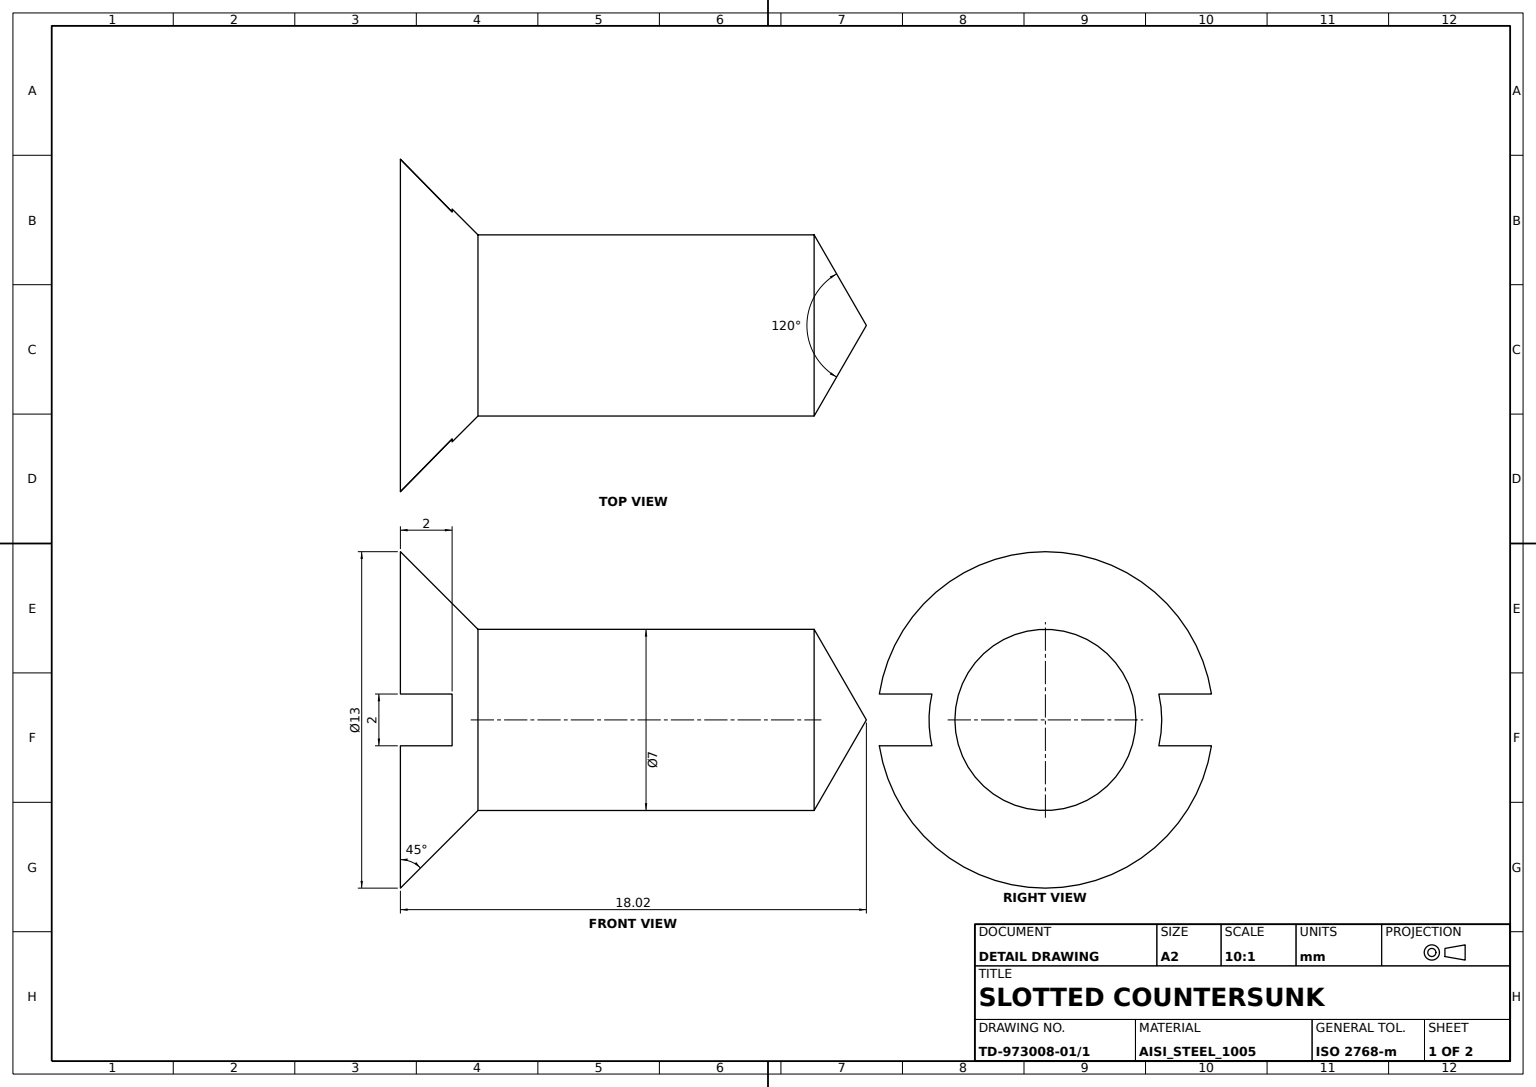
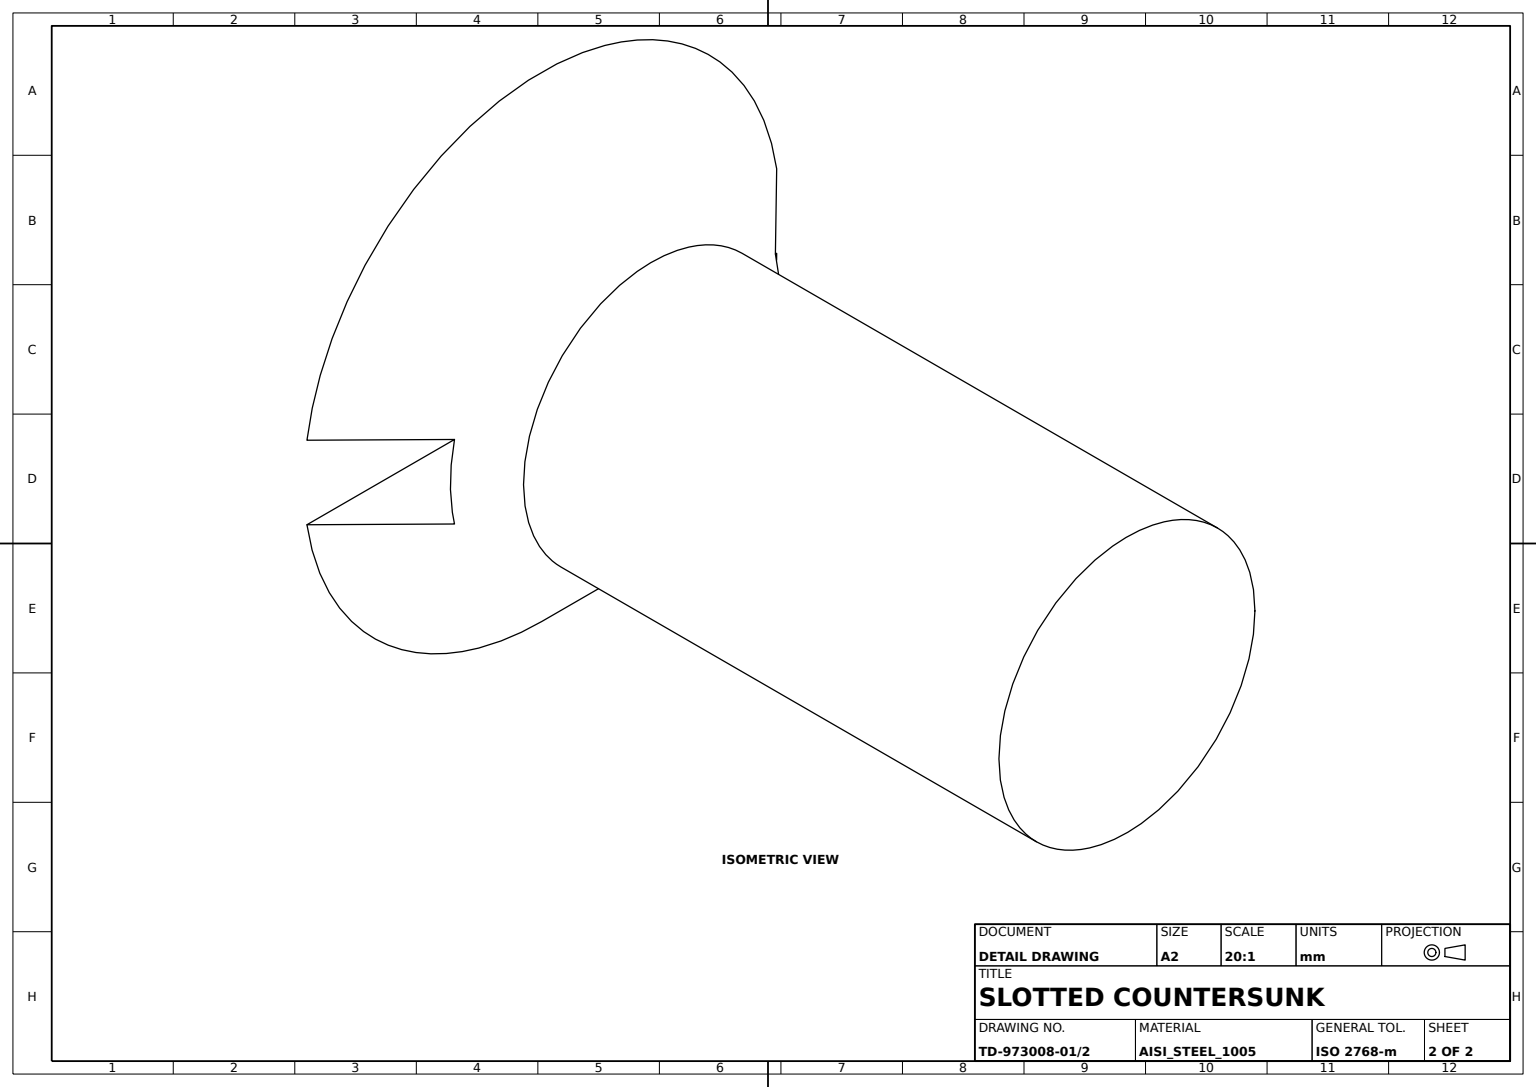
ISO-10303-21;
HEADER;
FILE_DESCRIPTION((''),'2;1');
FILE_NAME('','',(''),(''),'','','');
FILE_SCHEMA(('AUTOMOTIVE_DESIGN'));
ENDSEC;
DATA;
#1=APPLICATION_CONTEXT('');
#2=PRODUCT_CONTEXT('',#1,'mechanical');
#3=PRODUCT('','','',(#2));
#4=PRODUCT_DEFINITION_FORMATION('','',#3);
#5=PRODUCT_DEFINITION_CONTEXT('',#1,'design');
#6=PRODUCT_DEFINITION('','',#4,#5);
#7=PRODUCT_DEFINITION_SHAPE('','',#6);
#8=(LENGTH_UNIT()NAMED_UNIT(*)SI_UNIT(.MILLI.,.METRE.));
#9=(NAMED_UNIT(*)PLANE_ANGLE_UNIT()SI_UNIT($,.RADIAN.));
#10=(NAMED_UNIT(*)SI_UNIT($,.STERADIAN.)SOLID_ANGLE_UNIT());
#11=UNCERTAINTY_MEASURE_WITH_UNIT(LENGTH_MEASURE(0.005),#8,'distance_accuracy_value','');
#12=(GEOMETRIC_REPRESENTATION_CONTEXT(3)GLOBAL_UNCERTAINTY_ASSIGNED_CONTEXT((#11))GLOBAL_UNIT_ASSIGNED_CONTEXT((#8,#9,#10))REPRESENTATION_CONTEXT('',''));
#13=CARTESIAN_POINT('',(-17.425463,-1.,6.422616));
#14=VERTEX_POINT('',#13);
#15=CARTESIAN_POINT('',(-17.425463,-1.,-6.422616));
#16=VERTEX_POINT('',#15);
#17=CARTESIAN_POINT('',(-17.425463,-1.,7.));
#18=DIRECTION('',(0.,0.,-1.));
#19=VECTOR('',#18,1000.);
#20=LINE('',#17,#19);
#21=EDGE_CURVE('',#14,#16,#20,.T.);
#22=ORIENTED_EDGE('',*,*,#21,.T.);
#23=CARTESIAN_POINT('',(-17.425463,0.,0.));
#24=DIRECTION('',(1.,0.,0.));
#25=AXIS2_PLACEMENT_3D('',#23,#24,#18);
#26=CIRCLE('',#25,6.5);
#27=EDGE_CURVE('',#14,#16,#26,.T.);
#28=ORIENTED_EDGE('',*,*,#27,.F.);
#29=EDGE_LOOP('',(#22,#28));
#30=FACE_BOUND('',#29,.T.);
#31=CARTESIAN_POINT('',(-17.425463,6.5,0.));
#32=DIRECTION('',(-1.,0.,0.));
#33=DIRECTION('',(0.,0.,1.));
#34=AXIS2_PLACEMENT_3D('',#31,#32,#33);
#35=PLANE('',#34);
#36=ADVANCED_FACE('',(#30),#35,.T.);
#37=ORIENTED_EDGE('',*,*,#27,.T.);
#38=CARTESIAN_POINT('',(-15.425463,-1.,-4.387482));
#39=VERTEX_POINT('',#38);
#40=CARTESIAN_POINT('',(-16.089461,-1.,-5.068508));
#41=CARTESIAN_POINT('',(-16.756961,-1.,-5.746059));
#42=B_SPLINE_CURVE_WITH_KNOTS('',3,(#38,#40,#41,#15),.UNSPECIFIED.,.F.,.F.,(4,4),(0.025452548,0.028328148),.UNSPECIFIED.);
#43=EDGE_CURVE('',#39,#16,#42,.T.);
#44=ORIENTED_EDGE('',*,*,#43,.F.);
#45=CARTESIAN_POINT('',(-15.425463,1.,-4.387482));
#46=VERTEX_POINT('',#45);
#47=CARTESIAN_POINT('',(-15.425463,0.,0.));
#48=AXIS2_PLACEMENT_3D('',#47,#24,#18);
#49=CIRCLE('',#48,4.5);
#50=EDGE_CURVE('',#46,#39,#49,.F.);
#51=ORIENTED_EDGE('',*,*,#50,.F.);
#52=CARTESIAN_POINT('',(-17.425463,1.,-6.422616));
#53=VERTEX_POINT('',#52);
#54=CARTESIAN_POINT('',(-16.756955,1.,-5.746054));
#55=CARTESIAN_POINT('',(-16.089453,1.,-5.0685));
#56=B_SPLINE_CURVE_WITH_KNOTS('',3,(#52,#54,#55,#45),.UNSPECIFIED.,.F.,.F.,(4,4),(0.011190983,0.014044358),.UNSPECIFIED.);
#57=EDGE_CURVE('',#53,#46,#56,.T.);
#58=ORIENTED_EDGE('',*,*,#57,.F.);
#59=CARTESIAN_POINT('',(-17.425463,1.,6.422616));
#60=VERTEX_POINT('',#59);
#61=EDGE_CURVE('',#53,#60,#26,.T.);
#62=ORIENTED_EDGE('',*,*,#61,.T.);
#63=CARTESIAN_POINT('',(-15.425463,1.,4.387482));
#64=VERTEX_POINT('',#63);
#65=CARTESIAN_POINT('',(-16.089461,1.,5.068508));
#66=CARTESIAN_POINT('',(-16.756961,1.,5.746059));
#67=B_SPLINE_CURVE_WITH_KNOTS('',3,(#63,#65,#66,#59),.UNSPECIFIED.,.F.,.F.,(4,4),(0.025452548,0.028328148),.UNSPECIFIED.);
#68=EDGE_CURVE('',#64,#60,#67,.T.);
#69=ORIENTED_EDGE('',*,*,#68,.F.);
#70=CARTESIAN_POINT('',(-15.425463,-1.,4.387482));
#71=VERTEX_POINT('',#70);
#72=EDGE_CURVE('',#71,#64,#49,.F.);
#73=ORIENTED_EDGE('',*,*,#72,.F.);
#74=CARTESIAN_POINT('',(-16.756955,-1.,5.746054));
#75=CARTESIAN_POINT('',(-16.089453,-1.,5.0685));
#76=B_SPLINE_CURVE_WITH_KNOTS('',3,(#13,#74,#75,#70),.UNSPECIFIED.,.F.,.F.,(4,4),(0.011190983,0.014044358),.UNSPECIFIED.);
#77=EDGE_CURVE('',#14,#71,#76,.T.);
#78=ORIENTED_EDGE('',*,*,#77,.F.);
#79=EDGE_LOOP('',(#37,#44,#51,#58,#62,#69,#73,#78));
#80=FACE_BOUND('',#79,.T.);
#81=CARTESIAN_POINT('',(-14.425463,0.,-3.5));
#82=VERTEX_POINT('',#81);
#83=CARTESIAN_POINT('',(-14.425463,0.,0.));
#84=AXIS2_PLACEMENT_3D('',#83,#24,#18);
#85=CIRCLE('',#84,3.5);
#86=EDGE_CURVE('',#82,#82,#85,.T.);
#87=ORIENTED_EDGE('',*,*,#86,.F.);
#88=EDGE_LOOP('',(#87));
#89=FACE_BOUND('',#88,.T.);
#90=AXIS2_PLACEMENT_3D('',#83,#32,#33);
#91=CONICAL_SURFACE('',#90,3.5,0.785398163);
#92=ADVANCED_FACE('',(#80,#89),#91,.T.);
#93=ORIENTED_EDGE('',*,*,#21,.F.);
#94=ORIENTED_EDGE('',*,*,#77,.T.);
#95=CARTESIAN_POINT('',(-15.425463,-1.,7.));
#96=LINE('',#95,#19);
#97=EDGE_CURVE('',#39,#71,#96,.F.);
#98=ORIENTED_EDGE('',*,*,#97,.F.);
#99=ORIENTED_EDGE('',*,*,#43,.T.);
#100=EDGE_LOOP('',(#93,#94,#98,#99));
#101=FACE_BOUND('',#100,.T.);
#102=DIRECTION('',(0.,-1.,0.));
#103=AXIS2_PLACEMENT_3D('',#95,#102,#24);
#104=PLANE('',#103);
#105=ADVANCED_FACE('',(#101),#104,.F.);
#106=ORIENTED_EDGE('',*,*,#61,.F.);
#107=CARTESIAN_POINT('',(-17.425463,1.,7.));
#108=LINE('',#107,#19);
#109=EDGE_CURVE('',#60,#53,#108,.T.);
#110=ORIENTED_EDGE('',*,*,#109,.F.);
#111=EDGE_LOOP('',(#106,#110));
#112=FACE_BOUND('',#111,.T.);
#113=ADVANCED_FACE('',(#112),#35,.T.);
#114=ORIENTED_EDGE('',*,*,#50,.T.);
#115=ORIENTED_EDGE('',*,*,#97,.T.);
#116=ORIENTED_EDGE('',*,*,#72,.T.);
#117=CARTESIAN_POINT('',(-15.425463,1.,7.));
#118=LINE('',#117,#19);
#119=EDGE_CURVE('',#46,#64,#118,.F.);
#120=ORIENTED_EDGE('',*,*,#119,.F.);
#121=EDGE_LOOP('',(#114,#115,#116,#120));
#122=FACE_BOUND('',#121,.T.);
#123=AXIS2_PLACEMENT_3D('',#117,#24,#18);
#124=PLANE('',#123);
#125=ADVANCED_FACE('',(#122),#124,.F.);
#126=ORIENTED_EDGE('',*,*,#109,.T.);
#127=ORIENTED_EDGE('',*,*,#57,.T.);
#128=ORIENTED_EDGE('',*,*,#119,.T.);
#129=ORIENTED_EDGE('',*,*,#68,.T.);
#130=EDGE_LOOP('',(#126,#127,#128,#129));
#131=FACE_BOUND('',#130,.T.);
#132=DIRECTION('',(0.,1.,0.));
#133=AXIS2_PLACEMENT_3D('',#107,#132,#32);
#134=PLANE('',#133);
#135=ADVANCED_FACE('',(#131),#134,.F.);
#136=CARTESIAN_POINT('',(-1.425463,0.,-3.5));
#137=VERTEX_POINT('',#136);
#138=CARTESIAN_POINT('',(-1.425463,0.,0.));
#139=AXIS2_PLACEMENT_3D('',#138,#24,#18);
#140=CIRCLE('',#139,3.5);
#141=EDGE_CURVE('',#137,#137,#140,.T.);
#142=ORIENTED_EDGE('',*,*,#141,.F.);
#143=EDGE_LOOP('',(#142));
#144=FACE_BOUND('',#143,.T.);
#145=ORIENTED_EDGE('',*,*,#86,.T.);
#146=EDGE_LOOP('',(#145));
#147=FACE_BOUND('',#146,.T.);
#148=CARTESIAN_POINT('',(0.,0.,0.));
#149=AXIS2_PLACEMENT_3D('',#148,#24,#18);
#150=CYLINDRICAL_SURFACE('',#149,3.5);
#151=ADVANCED_FACE('',(#144,#147),#150,.T.);
#152=CARTESIAN_POINT('',(0.595263,0.,0.));
#153=VERTEX_POINT('',#152);
#154=VERTEX_LOOP('',#153);
#155=FACE_BOUND('',#154,.T.);
#156=ORIENTED_EDGE('',*,*,#141,.T.);
#157=EDGE_LOOP('',(#156));
#158=FACE_BOUND('',#157,.T.);
#159=AXIS2_PLACEMENT_3D('',#152,#32,#33);
#160=CONICAL_SURFACE('',#159,0.,1.047197551);
#161=ADVANCED_FACE('',(#155,#158),#160,.T.);
#162=CLOSED_SHELL('',(#36,#92,#105,#113,#125,#135,#151,#161));
#163=MANIFOLD_SOLID_BREP('',#162);
#164=ADVANCED_BREP_SHAPE_REPRESENTATION('',(#163),#12);
#165=SHAPE_DEFINITION_REPRESENTATION(#7,#164);
ENDSEC;
END-ISO-10303-21;
